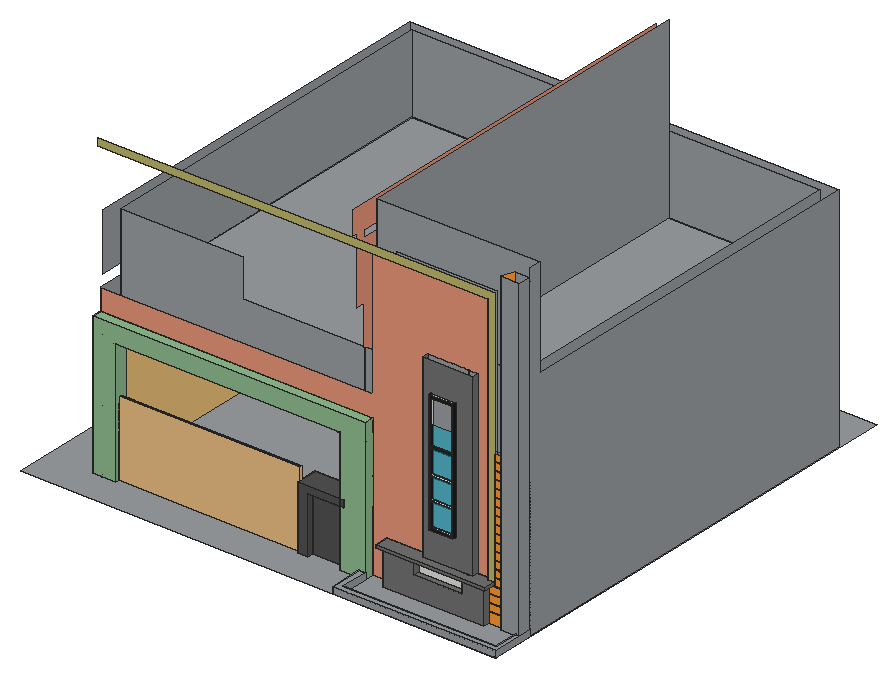
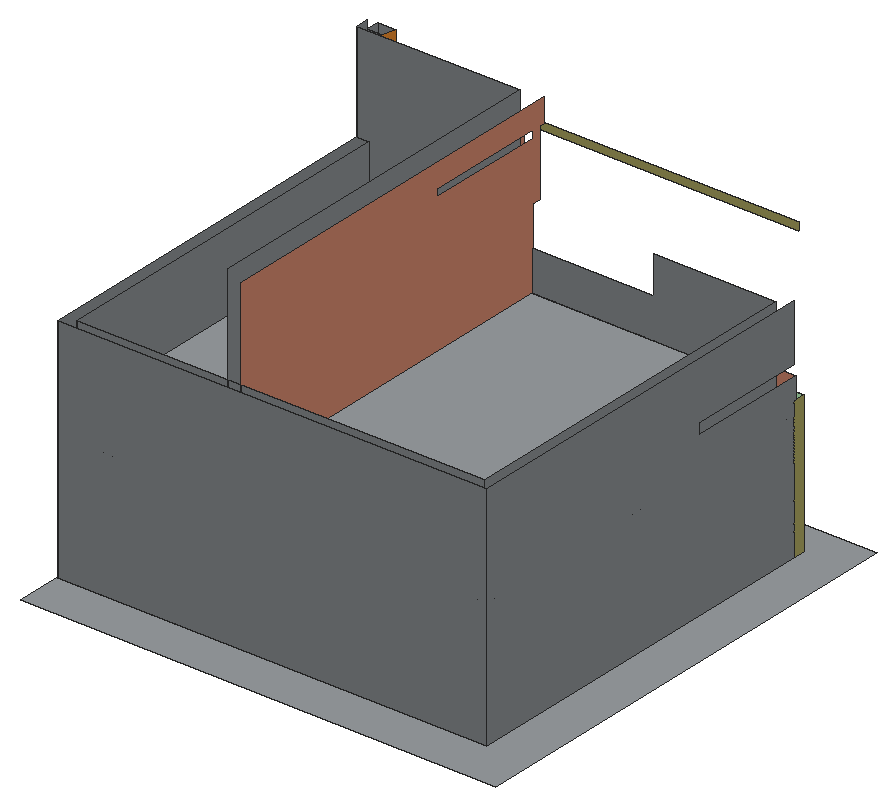
# SketchUp Ruby script. Lengths in inches.
U = 1.inch
M = Sketchup.active_model
def pt(a) = Geom::Point3d.new(a.map { |v| v * U })
def face(e, loops, mat)
  f = e.add_face(loops[0].map { |a| pt(a) })
  loops[1..].each { |l| e.add_face(l.map { |a| pt(a) }).erase! }
  f.material = f.back_material = mat if mat
  f
end
# faces: each face lists its corners as indices into pts; further lists are holes
def faces(e, pts, list, mat = nil) = list.each { |f| face(e, (f[0].is_a?(Array) ? f : [f]).map { |l| l.map { |i| pts[i] } }, mat) }
# xy, xz, yz: faces in a plane at the given z, y or x. An outline is a flat list of corners, or four numbers for a rectangle; further outlines are holes
def ring(l) = l.size == 4 ? [[l[0], l[1]], [l[2], l[1]], [l[2], l[3]], [l[0], l[3]]] : l.each_slice(2).to_a
def flat(e, list, mat, &to3) = list.each { |f| face(e, (f[0].is_a?(Array) ? f : [f]).map { |l| ring(l).map { |u, v| to3.(u, v) } }, mat) }
def xy(e, z, list, mat = nil) = flat(e, list, mat) { |x, y| [x, y, z] }
def xz(e, y, list, mat = nil) = flat(e, list, mat) { |x, z| [x, y, z] }
def yz(e, x, list, mat = nil) = flat(e, list, mat) { |y, z| [x, y, z] }
def lines(e, pts, list) = list.each { |a, b| e.add_line(pt(pts[a]), pt(pts[b])) }
# prism: a flat outline (further loops are holes) pulled along v
def prism(e, loops, v, mat = nil)
  f = face(e, loops, mat); d = Geom::Vector3d.new(v.map { |x| x * U })
  f.pushpull(f.normal.samedirection?(d) ? d.length : -d.length)
end
def box(e, o, s, mat = nil) = prism(e, [[o, [o[0] + s[0], o[1], o[2]], [o[0] + s[0], o[1] + s[1], o[2]], [o[0], o[1] + s[1], o[2]]]], [0, 0, s[2]], mat)
def at(x, y, z, deg = 0) = Geom::Transformation.translation(pt([x, y, z])) * Geom::Transformation.rotation(ORIGIN, Z_AXIS, deg.degrees)
def axes(o, x, y, z) = Geom::Transformation.new([*x, 0, *y, 0, *z, 0, *pt(o).to_a, 1])
def part(name) = M.definitions.add(name)
# library, detail: a bought-in or finely detailed component or shape, given as its bounding box
def library(name, o, s) = part(name).tap { |d| box(d.entities, o, s) }
def detail(e, o, s) = box(e.add_group.entities, o, s)
def put(e, d, t, mat = nil) = e.add_instance(d, t).tap { |i| i.material = mat if mat }
def group(e, t, mat = nil) = e.add_group.tap { |g| g.transformation = t; g.material = mat if mat }.entities
root = M.entities
M.materials.add("[0014_DarkSalmon]").color = [233, 150, 122]
M.materials.add("[0057_DarkKhaki]").color = [189, 183, 107]
M.materials.add("[0072_DarkSeaGreen]").color = [143, 188, 143]
M.materials.add("[0135_DarkGray]").color = [81, 81, 81]
M.materials.add("[Color A07]").color = [153, 0, 0]
M.materials.add("[Color C04]").color = [255, 153, 50]
M.materials.add("[Color M05]").color = [114, 114, 114]
M.materials.add("[Color M08]").color = [30, 30, 30]
M.materials.add("[Metal Rough]").color = [153, 157, 160]
M.materials.add("[Translucent Glass Gray]").color = [128, 128, 128]
M.materials["[Translucent Glass Gray]"].alpha = 0.5
M.materials.add("[Translucent Glass Tinted]").color = [8, 201, 241]
M.materials["[Translucent Glass Tinted]"].alpha = 0.48
M.materials.add("[Wood OSB]").color = [240, 195, 122]
M.materials.add("[Wood Veneer 01]").color = [120, 70, 37]
c1 = library("gate (1)",[0,0,0],[171.26,1.97,78.74])
xy(root,-0.125,[[52.17,31.17,61.96,31.79],[61.96,31.17,64.84,43.17],[52.17,31.79,61.96,43.17]],"[Metal Rough]")
xy(root,0,[[0,0,293.02,0,293.02,31.17,274.87,31.17,276.79,37.17,244.55,37.17,244.55,31.17,235.08,31.17,235.08,52.17,394.17,52.17,394.17,223.17,293.42,223.17,293.42,220.17,257.42,220.17,257.42,223.17,52.17,223.17,52.17,52.17,64.84,52.17,64.84,43.17,52.17,43.17,52.17,31.17,43.17,31.17,43.17,403.17,445.6,403.17,445.6,40.17,446.27,40.17,446.27,0,446.33,0,446.33,446.33,0,446.33],[293.02,0,445.71,1.42],[445.71,0,446.27,1.42],[293.02,1.42,293.02,31.17,298.9,31.17,298.9,5.26,442.39,5.26,442.39,40.17,445.71,40.17,445.71,1.42],[445.71,1.42,446.27,40.17],
  [298.9,5.26,442.39,5.26,442.39,40.17,410.18,40.17,410.18,31.17,315.29,31.17,315.29,40.17,298.9,40.17],[43.17,31.17,52.17,31.79],[235.08,31.17,244.55,43.17],[315.29,31.17,394.17,40.17],[394.17,31.17,410.18,40.17],
  [43.17,31.79,52.17,43.17],[244.55,37.17,276.79,37.17,278.71,43.17,244.55,43.17],[276.79,37.17,278.71,43.17,278.71,37.17],[394.17,40.17,394.17,394.17,52.17,394.17,52.17,43.17,43.17,43.17,43.17,403.17,445.6,403.17,445.6,40.42,410.18,40.42,410.18,40.17],[315.29,40.17,315.29,40.42,298.9,40.42,298.9,43.17,235.08,43.17,235.08,52.17,394.17,52.17,394.17,40.17],
  [298.9,40.17,315.29,40.42],[410.18,40.17,445.6,40.42],[52.17,43.17,64.84,52.17],[257.42,220.17,293.42,223.17],[52.17,223.17,394.17,232.58],
  [52.17,232.58,394.17,394.17]],"[Metal Rough]")
xy(root,0.03,[[405.02,37.17,432.3,40.17]],"[Metal Rough]")
xy(root,4.61,[[428.02,28.17,432.3,40.17,445.6,40.17,445.6,28.17]],"[Metal Rough]")
xy(root,6,[[293.02,0,446.27,0,446.27,40.17,442.39,40.17,442.39,5.26,298.9,5.26,298.9,31.17,293.02,31.17]],"[Metal Rough]")
xy(root,9.5,[[405.02,37.17,432.3,40.17]],"[Color C04]")
xy(root,10.41,[[401.77,37.17,415.14,40.17],[415.14,37.17,432.3,40.17]],"[Color C04]")
xy(root,17,[[401.77,37.17,432.3,40.17]],"[Color C04]")
xy(root,17.91,[[410.58,37.17,415.14,40.17],[415.14,37.17,432.3,40.17]],"[Color C04]")
xy(root,17.91,[[410.18,37.17,410.58,40.17]],"[Metal Rough]")
xy(root,20.28,[[344.57,31.17,389.01,36.85]],"[Color M05]")
xy(root,24.5,[[410.18,37.17,432.3,40.17]],"[Color C04]")
xy(root,24.77,[[126.14,220.17,229.57,223.17]],"[Color A07]")
xy(root,25.41,[[409.58,37.17,415.14,40.17],[415.14,37.17,432.3,40.17]],"[Color C04]")
xy(root,27.77,[[177.86,220.17,181.98,223.17]])
xy(root,27.77,[[129.14,220.17,177.86,223.17],[181.98,220.17,226.57,223.17]],"[Color A07]")
xy(root,30.78,[[344.57,31.17,389.01,36.85]],"[Color M05]")
xy(root,32,[[409.58,37.17,432.3,40.17]],"[Color C04]")
xy(root,32.91,[[415.14,37.17,432.3,40.17]],"[Color C04]")
xy(root,33.72,[[312.29,26.23,312.29,40.17,315.29,40.17,315.29,31.17,410.18,31.17,410.18,40.17,415.14,40.17,415.14,26.23]],"[Color M05]")
xy(root,33.72,[[312.29,40.17,315.29,40.42],[410.18,40.17,413.37,40.42]],"[Metal Rough]")
xy(root,36.3,[[312.29,26.23,415.14,26.23,415.14,37.17,409.48,37.17,411.24,40.17,396.98,40.17,396.98,34.17,393.23,34.17,393.23,34.1,389.11,34.1,389.11,34.17,350.73,34.17,350.73,40.17,312.29,40.17]],"[Color M05]")
xy(root,36.3,[[389.11,34.1,393.23,34.17],[350.73,34.17,396.98,40.17],[409.48,37.17,411.24,40.17,415.14,40.17,415.14,37.17],[312.29,40.17,350.73,40.42],[389.11,40.17,393.23,40.42],
  [393.23,40.17,413.37,40.42]],"[Metal Rough]")
xy(root,39.5,[[415.14,37.17,432.3,40.17]],"[Color C04]")
xy(root,40.41,[[415.14,37.17,432.3,40.17]],"[Color C04]")
xy(root,47,[[415.14,37.17,432.3,40.17]],"[Color C04]")
xy(root,47.91,[[415.14,37.17,432.3,40.17]],"[Color C04]")
xy(root,53.625,[[244.55,31.17,278.71,37.17]],"[0135_DarkGray]")
xy(root,53.625,[[244.55,37.17,274.02,43.17],[274.02,37.17,278.71,43.17]],"[Metal Rough]")
xy(root,54.5,[[415.14,37.17,432.3,40.17]],"[Color C04]")
xy(root,55.41,[[415.14,37.17,432.3,40.17]],"[Color C04]")
xy(root,60,[[235.08,31.17,278.71,31.17,278.71,43.17,298.9,43.17,298.9,45.73,394.17,45.73,394.17,52.17,235.08,52.17]],"[0135_DarkGray]")
xy(root,60,[[52.17,43.17,64.84,43.17,59.3125,52.17,52.17,52.17],[64.84,43.17,64.84,52.17,59.3125,52.17],[298.9,43.17,394.17,45.73]],"[Metal Rough]")
xy(root,62,[[415.14,37.17,432.3,40.17]],"[Color C04]")
xy(root,62.91,[[415.14,37.17,432.3,40.17]],"[Color C04]")
xy(root,63.14,[[358.25,31.17,381.3125,34.17]],"[Color M08]")
xy(root,64.86,[[359.96,31.17,379.6,34.17]])
xy(root,69.5,[[415.14,37.17,432.3,40.17]],"[Color C04]")
xy(root,70.41,[[415.14,37.17,432.3,40.17]],"[Color C04]")
xy(root,77,[[415.14,37.17,432.3,40.17]],"[Color C04]")
xy(root,77.91,[[415.14,37.17,432.3,40.17]],"[Color C04]")
xy(root,84,[[257.42,220.17,293.42,223.17]],"[Wood Veneer 01]")
xy(root,84.5,[[415.14,37.17,432.3,40.17]],"[Color C04]")
xy(root,85.41,[[415.14,37.17,432.3,40.17]],"[Color C04]")
xy(root,86.87,[[359.96,31.17,379.6,34.17]],"[Color M08]")
xy(root,87.88,[[359.96,31.17,379.6,34.17]])
xy(root,92,[[415.14,37.17,432.3,40.17]],"[Color C04]")
xy(root,92.91,[[415.14,37.17,432.3,40.17]],"[Color C04]")
xy(root,99.5,[[415.14,37.17,432.3,40.17]],"[Color C04]")
xy(root,100.41,[[415.14,37.17,432.3,40.17]],"[Color C04]")
xy(root,100.41,[[415.14,40.17,432.3,66.48],[415.14,66.48,432.3,70.48]],"[Metal Rough]")
xy(root,101.33,[[177.86,220.17,181.98,223.17]])
xy(root,101.33,[[129.14,220.17,177.86,223.17],[181.98,220.17,226.57,223.17]],"[Color A07]")
xy(root,104.33,[[126.14,220.17,229.57,223.17]],"[Color A07]")
xy(root,107,[[415.14,37.17,432.3,40.17]],"[Color C04]")
xy(root,107,[[415.14,40.17,432.3,66.48],[415.14,66.48,432.3,70.48]],"[Metal Rough]")
xy(root,107.91,[[415.14,37.17,432.3,40.17]],"[Color C04]")
xy(root,107.91,[[415.14,40.17,432.3,86.23]],"[Metal Rough]")
xy(root,108.05,[[359.96,31.17,379.6,34.17]],"[Color M08]")
xy(root,109.07,[[359.96,31.17,379.6,34.17]])
xy(root,114.5,[[415.14,37.17,432.3,40.17]],"[Color C04]")
xy(root,114.5,[[415.14,40.17,432.3,86.23]],"[Metal Rough]")
xy(root,115.41,[[415.14,37.17,432.3,40.17]],"[Color C04]")
xy(root,115.9,[[64.84,31.17,274.87,31.79],[274.87,31.17,274.87,31.79,275.07,31.79]])
xy(root,115.9,[[64.84,31.79,64.84,43.17,278.71,43.17,275.07,31.79]],"[0072_DarkSeaGreen]")
xy(root,115.9,[[61.96,31.79,64.84,43.17]],"[Metal Rough]")
xy(root,120,[[298.9,43.17,394.17,45.73],[52.17,223.17,394.17,232.58],[52.17,232.58,394.17,394.17]],"[Metal Rough]")
xy(root,120,[[52.17,43.17,52.17,223.17,394.17,223.17,394.17,45.73,298.9,45.73,298.9,43.17]],"[Wood OSB]")
xy(root,122,[[415.14,37.17,432.3,40.17]],"[Color C04]")
xy(root,122.91,[[415.14,37.17,432.3,40.17]],"[Color C04]")
xy(root,129.5,[[415.14,37.17,432.3,40.17]],"[Color C04]")
xy(root,130.41,[[415.14,37.17,432.3,40.17]],"[Color C04]")
xy(root,131.74,[[359.96,31.17,379.6,34.17]],"[Color M08]")
xy(root,132,[[43.17,31.17,298.9,40.17]],"[0072_DarkSeaGreen]")
xy(root,132,[[43.17,40.17,52.17,40.42],[52.17,40.17,298.9,40.42],[43.17,40.42,52.17,43.17],[52.17,40.42,298.9,43.17],[52.17,52.17,394.17,394.17]],"[Metal Rough]")
xy(root,132.76,[[359.96,31.17,379.6,34.17]],"[Color M08]")
xy(root,137,[[415.14,37.17,432.3,40.17]],"[Color C04]")
xy(root,137.91,[[415.14,37.17,432.3,40.17]],"[Color C04]")
xy(root,142.9375,[[52.17,52.17,281.37,394.17],[281.37,52.17,293.27,394.17],[293.27,52.17,434.73,394.17]],"[Metal Rough]")
xz(root,0,[[293.02,0,445.71,6],[445.71,0,446.27,6]],"[Metal Rough]")
xz(root,5.26,[[298.9,0,442.39,6]],"[Metal Rough]")
xz(root,26.23,[[312.29,33.72,415.14,36.3]],"[Color M05]")
xz(root,28.17,[[428.02,4.61,445.6,301.86]],"[Metal Rough]")
xz(root,31.17,[[52.17,-0.125,64.84,-0.125,64.84,115.9,274.87,115.9,274.87,60,278.71,60,278.71,53.625,274.87,53.625,274.87,0,293.02,0,293.02,6,298.9,6,298.9,132,43.17,132,43.17,0,52.17,0]],"[0072_DarkSeaGreen]")
xz(root,31.17,[[235.08,0,244.55,0,244.55,53.625,274.87,53.625,274.87,60,235.08,60],[274.87,53.625,278.71,60]],"[0135_DarkGray]")
xz(root,31.17,[[[315.29,0,410.18,33.72],[344.57,20.28,389.01,30.78]]],"[Color M05]")
xz(root,31.17,[[[358.25,63.14,381.3125,176.58],[359.96,64.86,379.6,174.87]],[359.96,86.87,379.6,87.88],[359.96,108.05,379.6,109.07],[359.96,131.74,379.6,132.76]],"[Color M08]")
xz(root,31.17,[[293.02,0,298.9,6]],"[Metal Rough]")
xz(root,34.17,[[[358.25,63.14,381.3125,176.58],[359.96,64.86,379.6,174.87]],[359.96,86.87,379.6,87.88],[359.96,108.05,379.6,109.07],[359.96,131.74,379.6,132.76]])
xz(root,34.17,[[[350.73,36.3,396.98,204.05],[358.25,63.14,381.3125,176.58]]],"[Color M05]")
xz(root,34.17,[[359.96,64.86,379.6,86.87],[359.96,87.88,379.6,108.05],[359.96,109.07,379.6,131.74],[359.96,132.76,379.6,150.37]],"[Translucent Glass Tinted]")
xz(root,36.85,[[344.57,20.28,389.01,30.78]])
xz(root,37.17,[[409.48,36.3,415.14,36.3,415.14,279.5,43.17,279.5,43.17,272.375,409.48,272.375]],"[0057_DarkKhaki]")
xz(root,37.17,[[244.55,0,278.71,53.625]],"[0135_DarkGray]")
xz(root,37.17,[[405.02,0.03,432.3,9.5],[401.77,10.41,432.3,17],[410.18,17.91,432.3,24.5],[409.58,25.41,432.3,32],[415.14,32.91,432.3,39.5],
  [415.14,40.41,432.3,47],[415.14,47.91,432.3,54.5],[415.14,55.41,432.3,62],[415.14,62.91,432.3,69.5],[415.14,70.41,432.3,77],
  [415.14,77.91,432.3,84.5],[415.14,85.41,432.3,92],[415.14,92.91,432.3,99.5],[415.14,100.41,432.3,107],[415.14,107.91,432.3,114.5],
  [415.14,115.41,432.3,122],[415.14,122.91,432.3,129.5],[415.14,130.41,432.3,137],[415.14,137.91,432.3,144.5]],"[Color C04]")
xz(root,40.17,[[298.9,0,315.29,0,315.29,33.72,312.29,33.72,312.29,36.3,350.73,36.3,350.73,204.05,396.98,204.05,396.98,36.3,411.24,36.3,411.24,272.375,298.9,272.375,298.9,152.08,43.17,152.08,43.17,132,298.9,132]],"[0014_DarkSalmon]")
xz(root,40.17,[[410.18,9.5,432.3,10.41],[410.18,24.5,432.3,25.41]],"[Color C04]")
xz(root,40.17,[[315.29,0,315.29,33.72,312.29,33.72,312.29,36.3,413.37,36.3,413.37,33.72,410.18,33.72,410.18,32,409.58,32,409.58,25.41,410.18,25.41,410.18,17,401.77,17,401.77,10.41,410.18,10.41,410.18,9.5,405.02,9.5,405.02,0.03,410.18,0.03,410.18,0],[410.18,0,442.39,0,442.39,4.61,432.3,4.61,432.3,0.03,410.18,0.03],[442.39,0,445.6,4.61],[445.6,0,446.27,6],[405.02,0.03,410.18,9.5],
  [410.18,0.03,415.14,9.5],[415.14,0.03,432.3,9.5],[432.3,4.61,442.39,4.61,442.39,6,445.6,6,445.6,301.86,432.3,301.86],[442.39,4.61,445.6,6],[401.77,10.41,410.18,17],
  [410.18,10.41,415.14,17],[415.14,10.41,432.3,17],[410.18,17,432.3,17.91],[410.18,17.91,410.58,24.5],[410.58,17.91,415.14,24.5],
  [415.14,17.91,432.3,24.5],[409.58,25.41,410.18,32],[410.18,25.41,415.14,32],[415.14,25.41,432.3,32],[410.18,32,432.3,32,432.3,32.91,415.14,32.91,415.14,33.72,410.18,33.72],
  [415.14,32.91,432.3,39.5],[413.37,33.72,415.14,36.3],[411.24,36.3,415.14,36.3,415.14,279.5,321.39,279.5,321.39,272.375,411.24,272.375],[350.73,36.3,389.11,204.05],[389.11,36.3,396.98,204.05],
  [415.14,39.5,432.3,40.41],[415.14,40.41,432.3,47],[415.14,47,432.3,47.91],[415.14,47.91,432.3,54.5],[415.14,54.5,432.3,55.41],
  [415.14,55.41,432.3,62],[415.14,62,432.3,62.91],[415.14,62.91,432.3,69.5],[415.14,69.5,432.3,70.41],[415.14,70.41,432.3,77],
  [415.14,77,432.3,77.91],[415.14,77.91,432.3,84.5],[415.14,84.5,432.3,85.41],[415.14,85.41,432.3,92],[415.14,92,432.3,92.91],
  [415.14,92.91,432.3,99.5],[415.14,99.5,432.3,100.41],[415.14,100.41,432.3,107],[415.14,107,432.3,107.91],[415.14,107.91,432.3,114.5],
  [415.14,114.5,432.3,115.41],[415.14,115.41,432.3,122],[415.14,122,432.3,122.91],[415.14,122.91,432.3,129.5],[415.14,129.5,432.3,130.41],
  [415.14,130.41,432.3,137],[415.14,137,432.3,137.91],[415.14,137.91,432.3,144.5]],"[Metal Rough]")
xz(root,43.17,[[52.17,-0.125,61.96,0],[61.96,-0.125,64.84,0],[43.17,0,52.17,1.75],[52.17,0,61.96,1.75],[61.96,0,64.84,1.75],
  [244.55,0,278.71,53.625],[278.71,0,298.9,60],[43.17,1.75,52.17,60],[52.17,1.75,61.96,60],[61.96,1.75,64.84,60],
  [43.17,60,52.17,132],[52.17,60,52.17,120,298.9,120,298.9,115.9,61.96,115.9,61.96,60],[61.96,60,64.84,115.9],[278.71,60,298.9,115.9],[298.9,60,394.17,120],
  [52.17,120,298.9,132],[298.9,132,438.67,216.1875]],"[Metal Rough]")
xz(root,45.73,[[298.9,60,394.17,120]],"[Metal Rough]")
xz(root,52.17,[[52.17,0,64.84,60],[235.08,0,394.17,60],[52.17,132,394.17,142.9375],[52.17,142.9375,52.17,216.1875,166.66,216.1875,166.66,180.82,281.37,180.82,281.37,142.9375],[281.37,142.9375,281.37,180.82,290.16,180.82,290.16,216.1875,293.27,216.1875,293.27,142.9375],
  [293.27,142.9375,293.27,309.37,445.6,309.37,445.6,216.1875,434.73,216.1875,434.73,142.9375]],"[Metal Rough]")
xz(root,66.48,[[415.14,100.41,432.3,107]],"[Metal Rough]")
xz(root,70.48,[[415.14,100.41,432.3,107]],"[Metal Rough]")
xz(root,86.23,[[415.14,107.91,432.3,114.5]],"[Metal Rough]")
xz(root,217.17,[[269.49,39.55,271.67,39.84,273.71,40.68,275.45,42.02,276.79,43.77,277.64,45.8,277.92,47.99,277.64,50.17,276.79,52.2,275.45,53.95,273.71,55.29,271.67,56.14,269.49,56.42,267.3,56.14,265.27,55.29,263.52,53.95,262.18,52.2,261.34,50.17,261.05,47.99,261.34,45.8,262.18,43.77,263.52,42.02,265.27,40.68,267.3,39.84]],"[Wood Veneer 01]")
xz(root,220.17,[[269.49,39.55,267.3,39.84,265.27,40.68,263.52,42.02,262.18,43.77,261.34,45.8,261.05,47.99,261.34,50.17,262.18,52.2,263.52,53.95,265.27,55.29,267.3,56.14,269.49,56.42,271.67,56.14,273.71,55.29,275.45,53.95,276.79,52.2,277.64,50.17,277.92,47.99,277.64,45.8,276.79,43.77,275.45,42.02,273.71,40.68,271.67,39.84]])
xz(root,220.17,[[[126.14,24.77,229.57,104.33],[129.14,27.77,226.57,101.33]],[177.86,27.77,181.98,101.33]],"[Color A07]")
xz(root,220.17,[[[257.42,0,293.42,84],[269.49,39.55,267.3,39.84,265.27,40.68,263.52,42.02,262.18,43.77,261.34,45.8,261.05,47.99,261.34,50.17,262.18,52.2,263.52,53.95,265.27,55.29,267.3,56.14,269.49,56.42,271.67,56.14,273.71,55.29,275.45,53.95,276.79,52.2,277.64,50.17,277.92,47.99,277.64,45.8,276.79,43.77,275.45,42.02,273.71,40.68,271.67,39.84]]],"[Wood Veneer 01]")
xz(root,223.17,[[[126.14,24.77,229.57,104.33],[129.14,27.77,226.57,101.33]],[177.86,27.77,181.98,101.33]])
xz(root,223.17,[[257.42,0,293.42,84]],"[Metal Rough]")
xz(root,223.17,[[129.14,27.77,177.86,101.33],[181.98,27.77,226.57,101.33]],"[Translucent Glass Gray]")
xz(root,223.17,[[[52.17,0,257.42,0,257.42,84,293.42,84,293.42,0,394.17,0,394.17,120,52.17,120],[126.14,24.77,229.57,104.33]]],"[Wood OSB]")
xz(root,232.58,[[52.17,0,394.17,120]],"[Metal Rough]")
xz(root,394.17,[[52.17,0,394.17,120],[52.17,132,394.17,142.9375],[52.17,142.9375,281.37,216.1875],[281.37,142.9375,293.27,216.1875],[293.27,142.9375,434.73,216.1875]],"[Metal Rough]")
xz(root,403.17,[[43.17,0,445.6,216.1875]],"[Metal Rough]")
yz(root,43.17,[[31.17,0,43.17,132]],"[0057_DarkKhaki]")
yz(root,43.17,[[43.17,0,43.17,132,40.42,132,40.42,152.08,154.25,152.08,154.25,162,43.17,162,43.17,216.1875,403.17,216.1875,403.17,0],[40.17,132,40.42,152.08]],"[Metal Rough]")
yz(root,52.17,[[31.17,-0.125,31.79,0],[31.79,-0.125,43.17,0],[43.17,0,52.17,60],[223.17,0,232.58,120],[232.58,0,394.17,120],
  [52.17,132,223.17,142.9375],[223.17,132,394.17,142.9375],[52.17,142.9375,394.17,216.1875]],"[Metal Rough]")
yz(root,52.17,[[52.17,0,223.17,0,223.17,120,43.17,120,43.17,60,52.17,60]],"[Wood OSB]")
yz(root,61.96,[[31.79,-0.125,43.17,115.9]],"[Metal Rough]")
yz(root,64.84,[[31.17,-0.125,43.17,115.9]],"[0072_DarkSeaGreen]")
yz(root,64.84,[[43.17,0,52.17,60]],"[Metal Rough]")
yz(root,126.14,[[220.17,24.77,223.17,104.33]],"[Color A07]")
yz(root,129.14,[[220.17,27.77,223.17,101.33]],"[Color A07]")
yz(root,177.86,[[220.17,27.77,223.17,101.33]],"[Color A07]")
yz(root,181.98,[[220.17,27.77,223.17,101.33]],"[Color A07]")
yz(root,226.57,[[220.17,27.77,223.17,101.33]],"[Color A07]")
yz(root,229.57,[[220.17,24.77,223.17,104.33]],"[Color A07]")
yz(root,235.08,[[31.17,0,52.17,60]],"[0135_DarkGray]")
yz(root,244.55,[[31.17,0,37.17,53.625]],"[0135_DarkGray]")
yz(root,244.55,[[37.17,0,43.17,53.625]],"[Metal Rough]")
yz(root,257.42,[[220.17,0,223.17,84]],"[Wood Veneer 01]")
yz(root,278.71,[[37.17,0,43.17,53.625],[31.17,53.625,43.17,60]],"[Metal Rough]")
yz(root,281.37,[[[52.17,142.9375,52.17,180.82,51.85,180.82,51.85,217.4375,43.17,217.4375,43.17,279.5,38.48,279.5,38.48,285.37,38.54,285.37,38.54,301.86,394.17,301.86,394.17,142.9375],[50.92,272.375,163.42,279.5]]],"[0014_DarkSalmon]")
yz(root,293.02,[[0,0,31.17,6]],"[Metal Rough]")
yz(root,293.27,[[52.17,142.9375,394.17,309.37]],"[Metal Rough]")
yz(root,293.42,[[220.17,0,223.17,84]],"[Wood Veneer 01]")
yz(root,298.9,[[31.17,0,40.17,132]],"[0072_DarkSeaGreen]")
yz(root,298.9,[[5.26,0,31.17,6],[40.17,0,40.42,60],[40.42,0,43.17,60],[40.17,60,40.42,120],[43.17,60,45.73,115.9],
  [43.17,115.9,45.73,120],[40.17,120,40.42,132],[40.42,120,43.17,132]],"[Metal Rough]")
yz(root,312.29,[[26.23,33.72,40.17,36.3]],"[Color M05]")
yz(root,312.29,[[40.17,33.72,40.42,36.3]],"[Metal Rough]")
yz(root,315.29,[[31.17,0,40.17,33.72]],"[Color M05]")
yz(root,315.29,[[40.17,0,40.42,33.72]],"[Metal Rough]")
yz(root,344.57,[[31.17,20.28,36.85,30.78]],"[Color M05]")
yz(root,350.73,[[34.17,36.3,40.17,204.05]],"[Color M05]")
yz(root,350.73,[[40.17,36.3,40.42,204.05]],"[Metal Rough]")
yz(root,358.25,[[31.17,63.14,34.17,176.58]],"[Color M08]")
yz(root,359.96,[[31.17,86.87,34.17,87.88],[31.17,108.05,34.17,109.07],[31.17,131.74,34.17,132.76]])
yz(root,359.96,[[31.17,64.86,34.17,86.87],[31.17,87.88,34.17,108.05],[31.17,109.07,34.17,131.74],[31.17,132.76,34.17,150.37]],"[Color M08]")
yz(root,379.6,[[31.17,86.87,34.17,87.88],[31.17,108.05,34.17,109.07],[31.17,131.74,34.17,132.76]])
yz(root,379.6,[[31.17,64.86,34.17,86.87],[31.17,87.88,34.17,108.05],[31.17,109.07,34.17,131.74],[31.17,132.76,34.17,150.37]],"[Color M08]")
yz(root,381.3125,[[31.17,63.14,34.17,176.58]],"[Color M08]")
yz(root,389.01,[[31.17,20.28,36.85,30.78]],"[Color M05]")
yz(root,389.11,[[40.17,36.3,40.42,204.05]],"[Metal Rough]")
yz(root,394.17,[[223.17,0,232.58,120],[232.58,0,394.17,120],[43.17,60,45.73,120]],"[Metal Rough]")
yz(root,394.17,[[52.17,0,52.17,60,45.73,60,45.73,120,223.17,120,223.17,0]],"[Wood OSB]")
yz(root,396.98,[[34.17,36.3,40.17,204.05]],"[Color M05]")
yz(root,401.77,[[37.17,10.41,40.17,17]],"[Metal Rough]")
yz(root,405.02,[[37.17,0.03,40.17,9.5]],"[Metal Rough]")
yz(root,409.58,[[37.17,25.41,40.17,32]],"[Metal Rough]")
yz(root,410.18,[[31.17,0,40.17,0,40.17,17.91,37.17,17.91,37.17,24.5,40.17,24.5,40.17,33.72,31.17,33.72]],"[Color M05]")
yz(root,410.18,[[40.17,0,40.42,33.72]],"[Metal Rough]")
yz(root,413.37,[[40.17,33.72,40.42,36.3]],"[Metal Rough]")
yz(root,415.14,[[26.23,33.72,37.17,36.3]],"[Color M05]")
yz(root,415.14,[[37.17,32.91,40.17,33.72],[37.17,33.72,40.17,36.3],[37.17,36.3,40.17,39.5],[37.17,39.5,40.17,40.41],[37.17,40.41,40.17,47],
  [37.17,47,40.17,47.91],[37.17,47.91,40.17,54.5],[37.17,54.5,40.17,55.41],[37.17,55.41,40.17,62],[37.17,62,40.17,62.91],
  [37.17,62.91,40.17,69.5],[37.17,69.5,40.17,70.41],[37.17,70.41,40.17,77],[37.17,77,40.17,77.91],[37.17,77.91,40.17,84.5],
  [37.17,84.5,40.17,85.41],[37.17,85.41,40.17,92],[37.17,92,40.17,92.91],[37.17,92.91,40.17,99.5],[37.17,99.5,40.17,100.41],
  [37.17,100.41,40.17,107],[40.17,100.41,66.48,107],[66.48,100.41,70.48,107],[37.17,107,40.17,107.91],[37.17,107.91,40.17,114.5],
  [40.17,107.91,86.23,114.5],[37.17,114.5,40.17,115.41],[37.17,115.41,40.17,122],[37.17,122,40.17,122.91],[37.17,122.91,40.17,129.5],
  [37.17,129.5,40.17,130.41],[37.17,130.41,40.17,137],[37.17,137,40.17,137.91],[37.17,137.91,40.17,144.5]],"[Metal Rough]")
yz(root,432.3,[[37.17,0.03,40.17,4.61],[37.17,4.61,40.17,9.5],[37.17,10.41,40.17,17],[37.17,17.91,40.17,24.5],[37.17,25.41,40.17,32],
  [37.17,32.91,40.17,39.5],[37.17,40.41,40.17,47],[37.17,47.91,40.17,54.5],[37.17,55.41,40.17,62],[37.17,62.91,40.17,69.5],
  [37.17,70.41,40.17,77],[37.17,77.91,40.17,84.5],[37.17,85.41,40.17,92],[37.17,92.91,40.17,99.5],[37.17,100.41,40.17,107],
  [40.17,100.41,66.48,107],[66.48,100.41,70.48,107],[37.17,107.91,40.17,114.5],[40.17,107.91,86.23,114.5],[37.17,115.41,40.17,122],
  [37.17,122.91,40.17,129.5],[37.17,130.41,40.17,137],[37.17,137.91,40.17,144.5]],"[Metal Rough]")
yz(root,434.73,[[52.17,142.9375,394.17,216.1875]],"[Metal Rough]")
yz(root,442.39,[[5.26,0,40.17,2.5],[5.26,2.5,40.17,6]],"[Metal Rough]")
yz(root,445.6,[[40.17,0,40.42,132],[40.42,0,403.17,0,403.17,216.1875,52.17,216.1875,52.17,309.37,40.42,309.37],[28.17,4.61,40.17,301.86],[40.17,132,40.42,216.1875]],"[Metal Rough]")
yz(root,446.27,[[0,0,40.17,6]],"[Metal Rough]")
p = [[274.87,31.17,115.9],[275.07,31.79,115.9],[278.71,43.17,115.9],[278.71,43.17,60],[278.71,43.17,53.625],[278.71,43.17,0],
  [276.79,37.17,0],[274.87,31.17,0],[274.87,31.17,53.625],[274.87,31.17,60],[428.02,28.17,301.86],[432.3,40.17,301.86],
  [432.3,40.17,279.5],[432.3,40.17,272.91],[432.3,40.17,272],[432.3,40.17,265.41],[432.3,40.17,264.5],[432.3,40.17,257.91],
  [432.3,40.17,257],[432.3,40.17,250.41],[432.3,40.17,249.5],[432.3,40.17,242.91],[432.3,40.17,242],[432.3,40.17,235.41],
  [432.3,40.17,234.5],[432.3,40.17,227.91],[432.3,40.17,227],[432.3,40.17,220.41],[432.3,40.17,219.5],[432.3,40.17,212.91],
  [432.3,40.17,212],[432.3,40.17,205.41],[432.3,40.17,204.5],[432.3,40.17,197.91],[432.3,40.17,197],[432.3,40.17,190.41],
  [432.3,40.17,189.5],[432.3,40.17,182.91],[432.3,40.17,182],[432.3,40.17,175.41],[432.3,40.17,174.5],[432.3,40.17,167.91],
  [432.3,40.17,167],[432.3,40.17,160.41],[432.3,40.17,159.5],[432.3,40.17,152.91],[432.3,40.17,152],[432.3,40.17,145.41],
  [432.3,40.17,144.5],[432.3,40.17,137.91],[432.3,40.17,137],[432.3,40.17,130.41],[432.3,40.17,129.5],[432.3,40.17,122.91],
  [432.3,40.17,122],[432.3,40.17,115.41],[432.3,40.17,114.5],[432.3,40.17,107.91],[432.3,40.17,107],[432.3,40.17,100.41],
  [432.3,40.17,99.5],[432.3,40.17,92.91],[432.3,40.17,92],[432.3,40.17,85.41],[432.3,40.17,84.5],[432.3,40.17,77.91],
  [432.3,40.17,77],[432.3,40.17,70.41],[432.3,40.17,69.5],[432.3,40.17,62.91],[432.3,40.17,62],[432.3,40.17,55.41],
  [432.3,40.17,54.5],[432.3,40.17,47.91],[432.3,40.17,47],[432.3,40.17,40.41],[432.3,40.17,39.5],[432.3,40.17,32.91],
  [432.3,40.17,32],[432.3,40.17,25.41],[432.3,40.17,24.5],[432.3,40.17,17.91],[432.3,40.17,17],[432.3,40.17,10.41],
  [432.3,40.17,9.5],[432.3,40.17,4.61],[428.02,28.17,4.61],[409.48,37.17,36.3],[409.48,37.17,272.375],[411.24,40.17,272.375],
  [411.24,40.17,36.3],[267.3,220.17,39.84],[269.49,220.17,39.55],[269.49,217.17,39.55],[267.3,217.17,39.84],[271.67,220.17,39.84],
  [271.67,217.17,39.84],[265.27,220.17,40.68],[265.27,217.17,40.68],[273.71,220.17,40.68],[273.71,217.17,40.68],[263.52,220.17,42.02],
  [263.52,217.17,42.02],[275.45,220.17,42.02],[275.45,217.17,42.02],[262.18,220.17,43.77],[262.18,217.17,43.77],[276.79,220.17,43.77],
  [276.79,217.17,43.77],[261.34,220.17,45.8],[261.34,217.17,45.8],[277.64,220.17,45.8],[277.64,217.17,45.8],[261.05,220.17,47.99],
  [261.05,217.17,47.99],[277.92,220.17,47.99],[277.92,217.17,47.99],[261.34,220.17,50.17],[261.34,217.17,50.17],[277.64,220.17,50.17],
  [277.64,217.17,50.17],[262.18,220.17,52.2],[262.18,217.17,52.2],[276.79,220.17,52.2],[276.79,217.17,52.2],[263.52,220.17,53.95],
  [263.52,217.17,53.95],[275.45,220.17,53.95],[275.45,217.17,53.95],[265.27,220.17,55.29],[265.27,217.17,55.29],[273.71,220.17,55.29],
  [273.71,217.17,55.29],[267.3,220.17,56.14],[267.3,217.17,56.14],[271.67,220.17,56.14],[271.67,217.17,56.14],[269.49,220.17,56.42],
  [269.49,217.17,56.42],[403.17,403.17,120],[403.17,394.17,120],[52.17,223.17,120],[52.17,223.17,132],[394.17,223.17,120],
  [394.17,223.17,132],[52.17,52.17,120],[43.17,52.17,120],[394.17,394.17,120],[394.17,403.17,120],[52.17,394.17,120],
  [52.17,403.17,120],[43.17,223.17,120],[43.17,394.17,120],[52.17,232.58,120],[43.17,232.58,120],[394.17,232.58,120],
  [403.17,232.58,120],[394.17,52.17,120],[403.17,52.17,120],[52.17,43.17,120],[52.17,31.17,120],[52.17,43.17,60],
  [52.17,31.17,60],[52.17,43.17,1.75],[52.17,31.17,1.75],[61.96,31.17,115.9],[61.96,31.79,115.9],[298.9,31.79,115.9],
  [394.17,223.17,142.9375],[438.67,43.17,132],[438.67,40.42,132],[274.02,43.17,60],[274.02,43.17,53.625],[442.39,5.26,2.5],
  [442.39,3.39,2.5]]
faces(root,p,[[0,1,2,3,4,5,6,7,8,9]],"[0072_DarkSeaGreen]")
faces(root,p,[[10,11,12,13,14,15,16,17,18,19,20,21,22,23,24,25,26,27,28,29,30,31,32,33,34,35,36,37,38,39,40,41,42,43,44,45,46,47,48,49,50,51,52,53,54,55,56,57,58,59,60,61,62,63,64,65,66,67,68,69,70,71,72,73,74,75,76,77,78,79,80,81,82,83,84,85,86]],"[Color C04]")
faces(root,p,[[87,88,89,90]],"[0057_DarkKhaki]")
faces(root,p,[[91,92,93,94],[92,95,96,93],[97,91,94,98],[95,99,100,96],[101,97,98,102],[99,103,104,100],[105,101,102,106],[103,107,108,104],
  [109,105,106,110],[107,111,112,108],[113,109,110,114],[111,115,116,112],[117,113,114,118],[115,119,120,116],[121,117,118,122],[119,123,124,120],
  [125,121,122,126],[123,127,128,124],[129,125,126,130],[127,131,132,128],[133,129,130,134],[131,135,136,132],[137,133,134,138],[135,137,138,136]],"[Wood Veneer 01]")
lines(root,p,[[139,140],[141,142],[143,144],[145,146],[147,148],[149,150],[141,151],[149,152],[153,154],[155,156],[147,140],[157,158],
  [159,160],[161,162],[163,164],[165,166],[1,167],[144,168],[169,170],[171,172],[173,174]])
put(root,c1,axes([64.84,34.48,0],[0.99407,0,0],[0,0.9,0],[0,0,0.9]))
